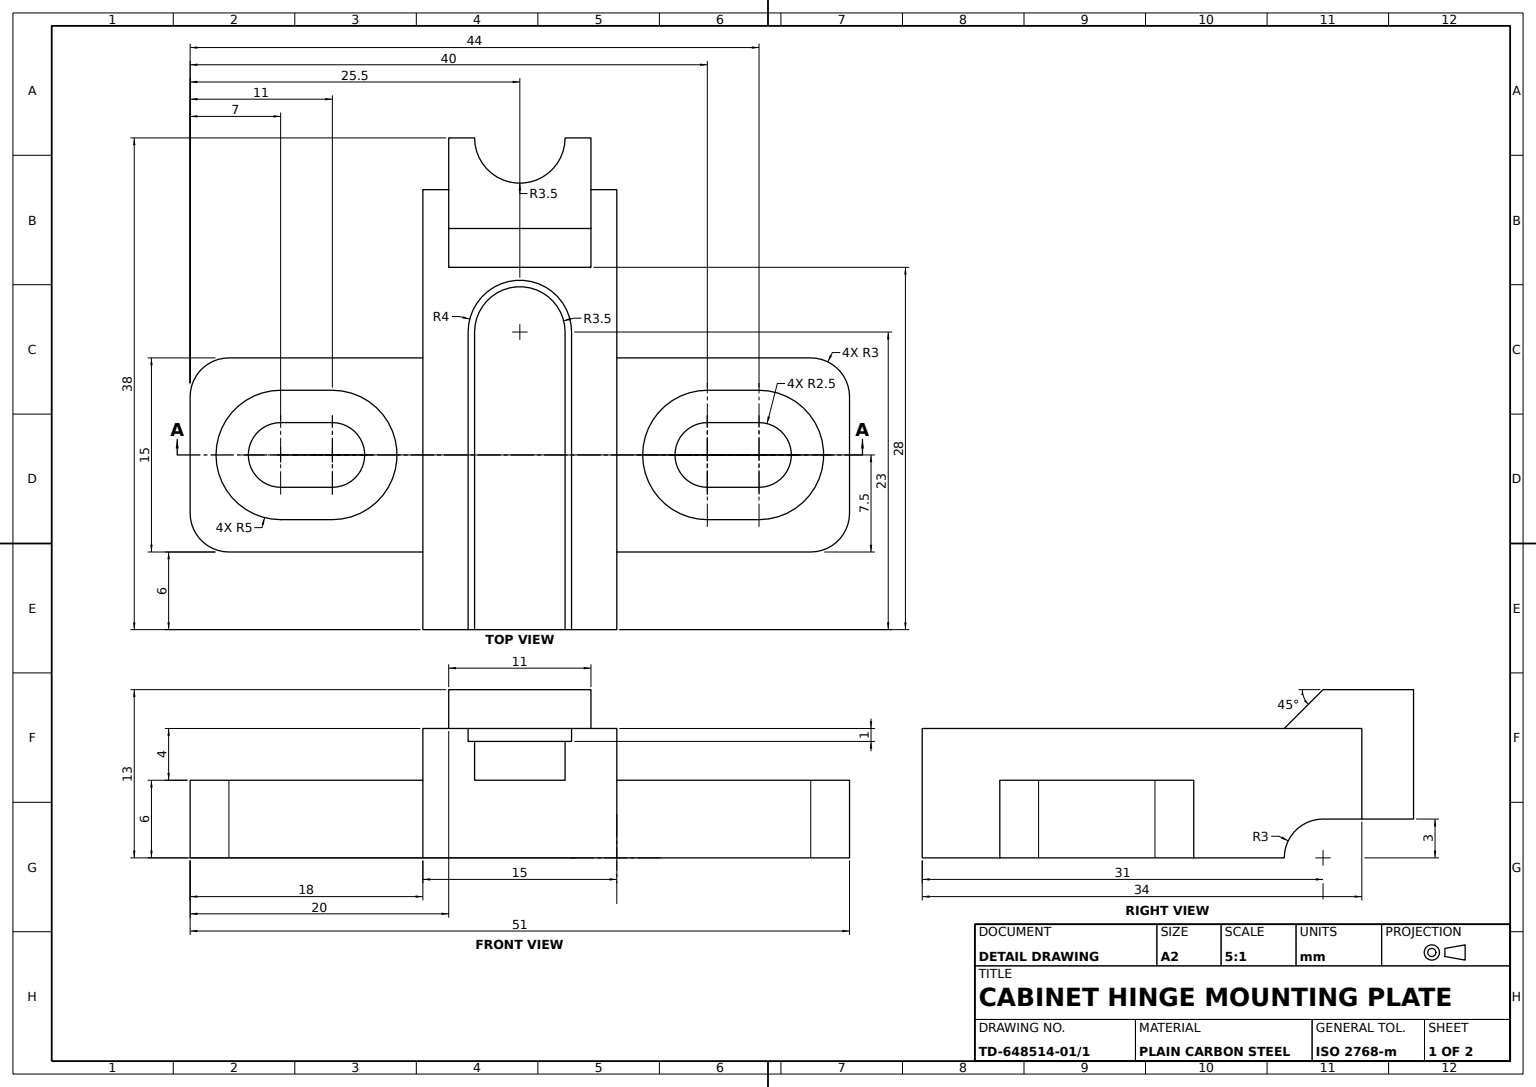
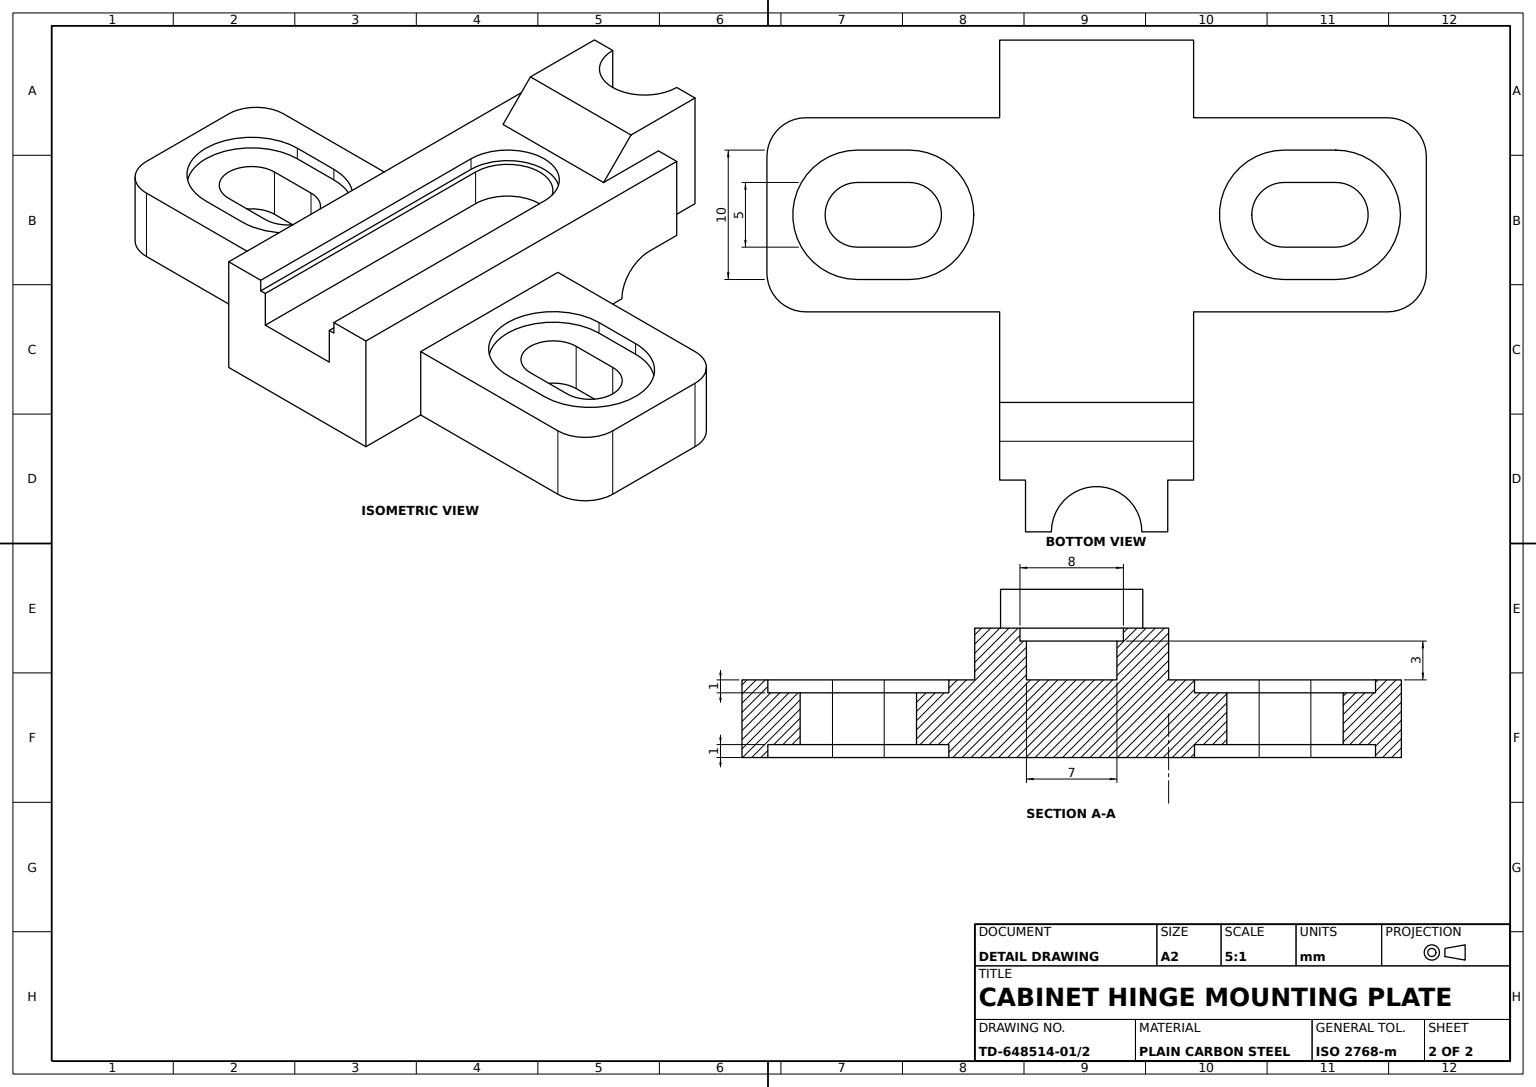
solid
v1 (-5,6,-18.5)
v2 (-5,6,-14.5)
e1 v1 v2 LINE
v3 (-5,5,-14.5)
e2 v3 v2 LINE
v4 (-5,5,-18.5)
e3 v4 v3 LINE
e4 v4 v1 LINE
face PLANE(AX(P(-5,5,-14.5),D(-1,0,0),D(0,0,1))) rev [e1 -e2 -e3 e4]
v5 (-24.5,13,-5.5)
v6 (-24.5,13,-3.5)
e5 v5 v6 LINE
v7 (-24.5,3,-5.5)
e6 v7 v5 LINE
v8 (-24.5,3,-3.5)
e7 v7 v8 LINE
e8 v8 v6 LINE
face PLANE(AX(P(-24.5,3,0),D(-1,0,0),D(0,0,1))) [-e5 -e6 e7 e8]
v9 (4.5,6,-25.5)
v10 (4.5,0,-25.5)
e9 v9 v10 LINE
v11 (-4.5,0,-25.5)
e10 v10 v11 LINE
v12 (-4.5,6,-25.5)
e11 v11 v12 LINE
e12 v9 v12 LINE
face PLANE(AX(P(-7.5,6,-25.5),D(0,0,1),D(1,0,0))) rev [e9 e10 e11 -e12]
v13 (-5,5,14.5)
v14 (5,5,14.5)
e13 v13 v14 CIRCLE(AX(P(0,5,14.5),D(0,-1,0),D(0,0,-1)),5)
v15 (5,6,14.5)
e14 v14 v15 LINE
v16 (-5,6,14.5)
e15 v16 v15 CIRCLE(AX(P(0,6,14.5),D(0,-1,0),D(0,0,-1)),5)
e16 v13 v16 LINE
face CYL(AX(P(0,5,14.5),D(0,1,0),D(0,0,1)),5) rev [e13 e14 -e15 -e16]
v17 (13.5,6,-3.5)
v18 (13.5,9,-3.5)
e17 v17 v18 LINE
v19 (13.5,6,3.5)
e18 v19 v17 LINE
v20 (13.5,9,3.5)
e19 v19 v20 LINE
v21 (13.5,9,4)
e20 v21 v20 LINE
v22 (13.5,10,4)
e21 v21 v22 LINE
v23 (13.5,10,7.5)
e22 v23 v22 LINE
v24 (13.5,0,7.5)
e23 v24 v23 LINE
v25 (13.5,0,-7.5)
e24 v24 v25 LINE
v26 (13.5,10,-7.5)
e25 v25 v26 LINE
v27 (13.5,10,-4)
e26 v27 v26 LINE
v28 (13.5,9,-4)
e27 v28 v27 LINE
e28 v18 v28 LINE
face PLANE(AX(P(13.5,0,7.5),D(1,0,0),D(0,0,-1))) [-e17 -e18 e19 -e20 e21 -e22 -e23 e24 e25 -e26 -e27 -e28]
v29 (-9.5,9,-3.5)
e29 v18 v29 LINE
v30 (-9.5,6,-3.5)
e30 v30 v29 LINE
e31 v17 v30 LINE
face PLANE(AX(P(-9.5,6,-3.5),D(0,0,-1),D(-1,0,0))) rev [e17 e29 -e30 -e31]
v31 (7.5,6,22.5)
v32 (7.5,6,7.5)
e32 v31 v32 LINE
v33 (7.5,0,22.5)
e33 v31 v33 LINE
v34 (7.5,0,7.5)
e34 v33 v34 LINE
e35 v34 v32 LINE
face PLANE(AX(P(7.5,6,-25.5),D(-1,0,0),D(0,0,1))) rev [-e32 e33 e34 e35]
v35 (5,1,-14.5)
v36 (5,0,-14.5)
e36 v35 v36 LINE
v37 (-5,0,-14.5)
e37 v37 v36 CIRCLE(AX(P(0,0,-14.5),D(0,1,0),D(0,0,1)),5)
v38 (-5,1,-14.5)
e38 v38 v37 LINE
e39 v38 v35 CIRCLE(AX(P(0,1,-14.5),D(0,1,0),D(0,0,1)),5)
face CYL(AX(P(0,1,-14.5),D(0,-1,0),D(0,0,-1)),5) rev [e36 -e37 -e38 e39]
v39 (-14.5,10,-5.5)
v40 (-14.5,10,5.5)
e40 v39 v40 LINE
v41 (-17.5,13,-5.5)
e41 v39 v41 LINE
v42 (-17.5,13,5.5)
e42 v41 v42 LINE
e43 v42 v40 LINE
face PLANE(AX(P(-17.5,13,-5.5),D(0.707106781,0.707106781,0),D(0,0,1))) [-e40 e41 e42 e43]
v43 (4.5,0,25.5)
e44 v33 v43 CIRCLE(AX(P(4.5,0,22.5),D(0,-1,0),D(0,0,-1)),3)
v44 (4.5,6,25.5)
e45 v44 v31 CIRCLE(AX(P(4.5,6,22.5),D(0,1,0),D(0,0,-1)),3)
e46 v43 v44 LINE
face CYL(AX(P(4.5,6,22.5),D(0,-1,0),D(0,0,-1)),3) [-e44 -e33 -e45 -e46]
v45 (0,5,-9.5)
v46 (5,5,-14.5)
e47 v45 v46 CIRCLE(AX(P(0,5,-14.5),D(0,1,0),D(0,0,1)),5)
v47 (5,5,-18.5)
e48 v46 v47 LINE
e49 v47 v4 CIRCLE(AX(P(0,5,-18.5),D(0,1,0),D(0,0,1)),5)
e50 v3 v45 CIRCLE(AX(P(0,5,-14.5),D(0,1,0),D(0,0,1)),5)
v48 (-2.5,5,-14.5)
v49 (0,5,-12)
e51 v48 v49 CIRCLE(AX(P(0,5,-14.5),D(0,1,0),D(0,0,1)),2.5)
v50 (-2.5,5,-18.5)
e52 v50 v48 LINE
v51 (2.5,5,-18.5)
e53 v51 v50 CIRCLE(AX(P(0,5,-18.5),D(0,1,0),D(0,0,1)),2.5)
v52 (2.5,5,-14.5)
e54 v52 v51 LINE
e55 v49 v52 CIRCLE(AX(P(0,5,-14.5),D(0,1,0),D(0,0,1)),2.5)
face PLANE(AX(P(0,5,-18.5),D(0,1,0),D(0,0,1))) [e47 e48 e49 e3 e50] [-e51 -e52 -e53 -e54 -e55]
v53 (-9.5,9,4)
e56 v53 v21 LINE
v54 (-9.5,9,3.5)
e57 v54 v20 LINE
e58 v29 v54 CIRCLE(AX(P(-9.5,9,0),D(0,1,0),D(0,0,1)),3.5)
v55 (-9.5,9,-4)
e59 v28 v55 LINE
e60 v55 v53 CIRCLE(AX(P(-9.5,9,0),D(0,1,0),D(0,0,1)),4)
face PLANE(AX(P(-9.5,9,0),D(0,1,0),D(0,0,1))) [e56 e20 -e57 -e58 -e29 e28 e59 e60]
v56 (5,6,18.5)
e61 v15 v56 LINE
v57 (0,6,23.5)
e62 v56 v57 CIRCLE(AX(P(0,6,18.5),D(0,-1,0),D(0,0,-1)),5)
v58 (-5,6,18.5)
e63 v57 v58 CIRCLE(AX(P(0,6,18.5),D(0,-1,0),D(0,0,-1)),5)
e64 v58 v16 LINE
v59 (-7.5,6,7.5)
e65 v32 v59 LINE
v60 (-7.5,6,22.5)
e66 v59 v60 LINE
v61 (-4.5,6,25.5)
e67 v60 v61 CIRCLE(AX(P(-4.5,6,22.5),D(0,1,0),D(0,0,-1)),3)
e68 v61 v44 LINE
face PLANE(AX(P(0,6,0),D(0,-1,0),D(0,0,-1))) rev [e15 e61 e62 e63 e64] [e32 e65 e66 e67 e68 e45]
v62 (-5,1,18.5)
v63 (-5,0,18.5)
e69 v62 v63 LINE
v64 (5,1,18.5)
e70 v64 v62 CIRCLE(AX(P(0,1,18.5),D(0,-1,0),D(0,0,-1)),5)
v65 (5,0,18.5)
e71 v64 v65 LINE
e72 v65 v63 CIRCLE(AX(P(0,0,18.5),D(0,-1,0),D(0,0,-1)),5)
face CYL(AX(P(0,1,18.5),D(0,-1,0),D(0,0,-1)),5) rev [-e69 -e70 e71 e72]
v66 (-5,5,18.5)
e73 v66 v58 LINE
v67 (0,5,23.5)
e74 v67 v57 LINE
e75 v67 v66 CIRCLE(AX(P(0,5,18.5),D(0,-1,0),D(0,0,-1)),5)
face CYL(AX(P(0,5,18.5),D(0,1,0),D(0,0,1)),5) rev [e73 -e63 -e74 e75]
v68 (-7.5,0,-22.5)
e76 v68 v11 CIRCLE(AX(P(-4.5,0,-22.5),D(0,-1,0),D(0,0,-1)),3)
v69 (-7.5,6,-22.5)
e77 v69 v68 LINE
e78 v12 v69 CIRCLE(AX(P(-4.5,6,-22.5),D(0,1,0),D(0,0,-1)),3)
face CYL(AX(P(-4.5,6,-22.5),D(0,-1,0),D(0,0,-1)),3) [-e11 -e76 -e77 -e78]
v70 (7.5,6,-22.5)
e79 v70 v9 CIRCLE(AX(P(4.5,6,-22.5),D(0,1,0),D(0,0,-1)),3)
v71 (-7.5,6,-7.5)
e80 v69 v71 LINE
v72 (7.5,6,-7.5)
e81 v71 v72 LINE
e82 v72 v70 LINE
v73 (5,6,-18.5)
e83 v73 v1 CIRCLE(AX(P(0,6,-18.5),D(0,1,0),D(0,0,1)),5)
v74 (5,6,-14.5)
e84 v74 v73 LINE
v75 (0,6,-9.5)
e85 v75 v74 CIRCLE(AX(P(0,6,-14.5),D(0,1,0),D(0,0,1)),5)
e86 v2 v75 CIRCLE(AX(P(0,6,-14.5),D(0,1,0),D(0,0,1)),5)
face PLANE(AX(P(0,6,0),D(0,-1,0),D(0,0,-1))) rev [e79 e12 e78 e80 e81 e82] [-e1 -e83 -e84 -e85 -e86]
v76 (-24.5,3,3.5)
e87 v76 v8 CIRCLE(AX(P(-24.5,3,0),D(0,1,0),D(0,0,1)),3.5)
v77 (-24.5,13,3.5)
e88 v76 v77 LINE
e89 v77 v6 CIRCLE(AX(P(-24.5,13,0),D(0,1,0),D(0,0,1)),3.5)
face CYL(AX(P(-24.5,3,0),D(0,1,0),D(0,0,1)),3.5) rev [-e87 e88 e89 -e8]
v78 (5,1,14.5)
e90 v78 v64 LINE
v79 (5,0,14.5)
e91 v78 v79 LINE
e92 v79 v65 LINE
face PLANE(AX(P(5,1,14.5),D(1,0,0),D(0,0,-1))) rev [-e90 e91 e92 -e71]
v80 (-4.5,0,25.5)
e93 v61 v80 LINE
e94 v80 v43 LINE
face PLANE(AX(P(7.5,6,25.5),D(0,0,-1),D(-1,0,0))) rev [e46 -e68 e93 e94]
v81 (7.5,0,-7.5)
v82 (7.5,0,-22.5)
e95 v81 v82 LINE
e96 v82 v70 LINE
e97 v72 v81 LINE
face PLANE(AX(P(7.5,6,-25.5),D(-1,0,0),D(0,0,1))) rev [e95 e96 -e82 e97]
v83 (-20.5,10,-7.5)
v84 (-20.5,10,-5.5)
e98 v83 v84 LINE
v85 (-20.5,3,-7.5)
e99 v85 v83 LINE
v86 (-20.5,3,-5.5)
e100 v85 v86 LINE
e101 v86 v84 LINE
face PLANE(AX(P(-20.5,0,0),D(-1,0,0),D(0,0,1))) [-e98 -e99 e100 e101]
v87 (-5,1,-18.5)
e102 v87 v38 LINE
v88 (0,1,-23.5)
e103 v88 v87 CIRCLE(AX(P(0,1,-18.5),D(0,1,0),D(0,0,1)),5)
v89 (5,1,-18.5)
e104 v89 v88 CIRCLE(AX(P(0,1,-18.5),D(0,1,0),D(0,0,1)),5)
e105 v35 v89 LINE
v90 (2.5,1,-14.5)
v91 (2.5,1,-18.5)
e106 v90 v91 LINE
v92 (-2.5,1,-18.5)
e107 v91 v92 CIRCLE(AX(P(0,1,-18.5),D(0,1,0),D(0,0,-1)),2.5)
v93 (-2.5,1,-14.5)
e108 v92 v93 LINE
v94 (0,1,-12)
e109 v93 v94 CIRCLE(AX(P(0,1,-14.5),D(0,1,0),D(0,0,-1)),2.5)
e110 v94 v90 CIRCLE(AX(P(0,1,-14.5),D(0,1,0),D(0,0,-1)),2.5)
face PLANE(AX(P(0,1,-18.5),D(0,-1,0),D(0,0,1))) [-e102 -e103 -e104 -e105 -e39] [e106 e107 e108 e109 e110]
v95 (5,5,18.5)
e111 v95 v56 LINE
e112 v95 v67 CIRCLE(AX(P(0,5,18.5),D(0,-1,0),D(0,0,-1)),5)
face CYL(AX(P(0,5,18.5),D(0,1,0),D(0,0,1)),5) rev [-e111 e112 e74 -e62]
e113 v90 v52 LINE
e114 v91 v51 LINE
face PLANE(AX(P(2.5,-6,-18.5),D(1,0,0),D(0,0,-1))) rev [-e106 e113 e54 -e114]
v96 (-7.5,0,7.5)
e115 v59 v96 LINE
e116 v34 v24 LINE
v97 (-20.5,10,7.5)
e117 v97 v23 LINE
v98 (-20.5,3,7.5)
e118 v98 v97 LINE
v99 (-17.5,3,7.5)
e119 v99 v98 LINE
v100 (-14.5,0,7.5)
e120 v99 v100 CIRCLE(AX(P(-17.5,0,7.5),D(0,0,-1),D(1,0,0)),3)
e121 v100 v96 LINE
face PLANE(AX(P(-9.5,0,7.5),D(0,0,1),D(1,0,0))) [-e115 -e65 -e35 e116 e23 -e117 -e118 -e119 e120 e121]
v101 (-9.5,6,3.5)
e122 v30 v101 CIRCLE(AX(P(-9.5,6,0),D(0,1,0),D(0,0,1)),3.5)
e123 v101 v19 LINE
face PLANE(AX(P(-9.5,6,0),D(0,1,0),D(0,0,1))) [e18 e31 e122 e123]
e124 v66 v13 LINE
face PLANE(AX(P(-5,5,14.5),D(1,0,0),D(0,0,-1))) [e16 -e64 -e73 e124]
e125 v47 v73 LINE
face CYL(AX(P(0,5,-18.5),D(0,1,0),D(0,0,1)),5) rev [-e4 -e49 e125 e83]
v102 (0,0,-23.5)
v103 (-5,0,-18.5)
e126 v102 v103 CIRCLE(AX(P(0,0,-18.5),D(0,1,0),D(0,0,1)),5)
e127 v88 v102 LINE
e128 v87 v103 LINE
face CYL(AX(P(0,1,-18.5),D(0,-1,0),D(0,0,-1)),5) rev [-e126 -e127 e103 e128]
v104 (0,1,21)
v105 (-2.5,1,18.5)
e129 v104 v105 CIRCLE(AX(P(0,1,18.5),D(0,-1,0),D(0,0,-1)),2.5)
v106 (-2.5,5,18.5)
e130 v105 v106 LINE
v107 (0,5,21)
e131 v106 v107 CIRCLE(AX(P(0,5,18.5),D(0,1,0),D(0,0,1)),2.5)
e132 v104 v107 LINE
face CYL(AX(P(0,-6,18.5),D(0,1,0),D(0,0,1)),2.5) rev [e129 e130 e131 -e132]
e133 v45 v75 LINE
face CYL(AX(P(0,5,-14.5),D(0,1,0),D(0,0,1)),5) rev [e2 e86 -e133 -e50]
v108 (5,0,-18.5)
e134 v36 v108 LINE
e135 v108 v102 CIRCLE(AX(P(0,0,-18.5),D(0,1,0),D(0,0,1)),5)
e136 v103 v37 LINE
v109 (0,0,9.5)
e137 v109 v79 CIRCLE(AX(P(0,0,14.5),D(0,-1,0),D(0,0,-1)),5)
v110 (-5,0,14.5)
e138 v110 v109 CIRCLE(AX(P(0,0,14.5),D(0,-1,0),D(0,0,-1)),5)
e139 v63 v110 LINE
v111 (-7.5,0,22.5)
e140 v96 v111 LINE
v112 (-14.5,0,-7.5)
e141 v112 v100 LINE
v113 (-7.5,0,-7.5)
e142 v113 v112 LINE
e143 v68 v113 LINE
e144 v10 v82 CIRCLE(AX(P(4.5,0,-22.5),D(0,-1,0),D(0,0,-1)),3)
e145 v25 v81 LINE
e146 v80 v111 CIRCLE(AX(P(-4.5,0,22.5),D(0,-1,0),D(0,0,-1)),3)
face PLANE(AX(P(0,0,0),D(0,-1,0),D(0,0,-1))) [e134 e135 e126 e136 e37] [-e72 -e92 -e137 -e138 -e139] [-e140 -e121 -e141 -e142 -e143 e76 -e10 e144 -e95 -e145 -e24 -e116 -e34 e44 -e94 e146]
v114 (-24.5,3,5.5)
e147 v76 v114 LINE
v115 (-24.5,13,5.5)
e148 v114 v115 LINE
e149 v77 v115 LINE
face PLANE(AX(P(-24.5,3,0),D(-1,0,0),D(0,0,1))) [-e88 e147 e148 -e149]
v116 (-2.5,1,14.5)
v117 (2.5,1,14.5)
e150 v116 v117 CIRCLE(AX(P(0,1,14.5),D(0,-1,0),D(0,0,-1)),2.5)
v118 (2.5,5,14.5)
e151 v117 v118 LINE
v119 (-2.5,5,14.5)
e152 v118 v119 CIRCLE(AX(P(0,5,14.5),D(0,1,0),D(0,0,1)),2.5)
e153 v116 v119 LINE
face CYL(AX(P(0,-6,14.5),D(0,1,0),D(0,0,1)),2.5) rev [e150 e151 e152 -e153]
v120 (-17.5,3,-7.5)
e154 v85 v120 LINE
e155 v120 v99 LINE
v121 (-20.5,3,5.5)
e156 v121 v98 LINE
e157 v114 v121 LINE
e158 v86 v7 LINE
face PLANE(AX(P(0,3,0),D(0,1,0),D(0,0,1))) rev [-e100 e154 e155 e119 -e156 -e157 -e147 e87 -e7 -e158]
e159 v46 v74 LINE
face PLANE(AX(P(5,5,-14.5),D(1,0,0),D(0,0,-1))) rev [e84 -e125 -e48 e159]
e160 v41 v5 LINE
e161 v84 v39 LINE
face PLANE(AX(P(0,3,-5.5),D(0,0,-1),D(-1,0,0))) [-e160 -e41 -e161 -e101 e158 e6]
v122 (0,1,9.5)
e162 v122 v78 CIRCLE(AX(P(0,1,14.5),D(0,-1,0),D(0,0,-1)),5)
e163 v122 v109 LINE
face CYL(AX(P(0,1,14.5),D(0,-1,0),D(0,0,-1)),5) rev [-e91 -e162 e163 e137]
face PLANE(AX(P(-5,1,-14.5),D(1,0,0),D(0,0,-1))) [-e128 e102 e38 -e136]
v123 (2.5,1,18.5)
e164 v123 v104 CIRCLE(AX(P(0,1,18.5),D(0,-1,0),D(0,0,-1)),2.5)
e165 v117 v123 LINE
e166 v105 v116 LINE
v124 (-5,1,14.5)
e167 v62 v124 LINE
e168 v124 v122 CIRCLE(AX(P(0,1,14.5),D(0,-1,0),D(0,0,-1)),5)
face PLANE(AX(P(0,1,18.5),D(0,-1,0),D(0,0,-1))) [-e129 -e164 -e165 -e150 -e166] [e162 e90 e70 e167 e168]
e169 v94 v49 LINE
face CYL(AX(P(0,-6,-14.5),D(0,1,0),D(0,0,1)),2.5) rev [-e113 -e110 e169 e55]
e170 v92 v50 LINE
face CYL(AX(P(0,-6,-18.5),D(0,1,0),D(0,0,1)),2.5) rev [e53 -e170 -e107 e114]
e171 v112 v120 CIRCLE(AX(P(-17.5,0,-7.5),D(0,0,1),D(-1,0,0)),3)
face CYL(AX(P(-17.5,0,0),D(0,0,-1),D(-1,0,0)),3) rev [-e171 e141 -e120 -e155]
e172 v124 v110 LINE
face PLANE(AX(P(-5,1,14.5),D(-1,0,0),D(0,0,1))) rev [e139 -e172 -e167 e69]
e173 v14 v95 LINE
face PLANE(AX(P(5,5,14.5),D(-1,0,0),D(0,0,1))) [-e61 -e14 e173 e111]
e174 v93 v48 LINE
face CYL(AX(P(0,-6,-14.5),D(0,1,0),D(0,0,1)),2.5) rev [-e109 e174 e51 -e169]
v125 (2.5,5,18.5)
e175 v107 v125 CIRCLE(AX(P(0,5,18.5),D(0,1,0),D(0,0,1)),2.5)
e176 v119 v106 LINE
e177 v125 v118 LINE
face PLANE(AX(P(0,5,18.5),D(0,1,0),D(0,0,-1))) [-e124 -e75 -e112 -e173 -e13] [-e175 -e131 -e176 -e152 -e177]
face PLANE(AX(P(-2.5,-6,14.5),D(-1,0,0),D(0,0,1))) rev [-e130 e166 e153 e176]
face CYL(AX(P(4.5,6,-22.5),D(0,-1,0),D(0,0,-1)),3) [-e9 -e79 -e96 -e144]
e178 v101 v54 LINE
face PLANE(AX(P(13.5,6,3.5),D(0,0,1),D(1,0,0))) rev [-e19 -e123 e178 e57]
face CYL(AX(P(0,1,14.5),D(0,-1,0),D(0,0,-1)),5) rev [e138 -e163 -e168 e172]
v126 (-9.5,10,4)
e179 v126 v22 LINE
e180 v53 v126 LINE
face PLANE(AX(P(13.5,9,4),D(0,0,1),D(1,0,0))) rev [e179 -e21 -e56 e180]
e181 v113 v71 LINE
e182 v26 v83 LINE
face PLANE(AX(P(13.5,0,-7.5),D(0,0,-1),D(-1,0,0))) [e145 -e97 -e81 -e181 e142 e171 -e154 e99 -e182 -e25]
e183 v115 v42 LINE
face PLANE(AX(P(0,13,0),D(0,1,0),D(0,0,1))) [-e42 e160 e5 -e89 e149 e183]
e184 v111 v60 LINE
face CYL(AX(P(-4.5,6,22.5),D(0,-1,0),D(0,0,-1)),3) [-e93 -e67 -e184 -e146]
v127 (-20.5,10,5.5)
e185 v127 v40 LINE
e186 v121 v127 LINE
face PLANE(AX(P(0,3,5.5),D(0,0,1),D(1,0,0))) [e185 -e43 -e183 -e148 e157 e186]
e187 v89 v108 LINE
face CYL(AX(P(0,1,-18.5),D(0,-1,0),D(0,0,-1)),5) rev [-e187 e104 e127 -e135]
v128 (-9.5,10,-4)
e188 v55 v128 LINE
e189 v128 v126 CIRCLE(AX(P(-9.5,10,0),D(0,1,0),D(0,0,1)),4)
face CYL(AX(P(-9.5,9,0),D(0,1,0),D(0,0,1)),4) rev [-e60 e188 e189 -e180]
face PLANE(AX(P(-7.5,6,0),D(1,0,0),D(0,0,-1))) rev [e77 e143 e181 -e80]
e190 v123 v125 LINE
face CYL(AX(P(0,-6,18.5),D(0,1,0),D(0,0,1)),2.5) rev [e175 -e190 e164 e132]
face PLANE(AX(P(-2.5,-6,-18.5),D(-1,0,0),D(0,0,1))) rev [-e174 -e108 e170 e52]
face PLANE(AX(P(-7.5,6,0),D(1,0,0),D(0,0,-1))) rev [e140 e184 -e66 e115]
face CYL(AX(P(-9.5,6,0),D(0,1,0),D(0,0,1)),3.5) rev [e30 e58 -e178 -e122]
face PLANE(AX(P(5,1,-14.5),D(-1,0,0),D(0,0,1))) [-e36 e105 e187 -e134]
face CYL(AX(P(0,5,-14.5),D(0,1,0),D(0,0,1)),5) rev [-e159 -e47 e133 e85]
e191 v27 v128 LINE
e192 v127 v97 LINE
face PLANE(AX(P(0,10,0),D(0,1,0),D(0,0,1))) [-e191 e26 e182 e98 e161 e40 -e185 e192 e117 e22 -e179 -e189]
face PLANE(AX(P(-9.5,9,-4),D(0,0,-1),D(-1,0,0))) rev [-e188 -e59 e27 e191]
face PLANE(AX(P(2.5,-6,14.5),D(1,0,0),D(0,0,-1))) rev [e177 -e151 e165 e190]
face PLANE(AX(P(-20.5,0,0),D(-1,0,0),D(0,0,1))) [-e186 e156 e118 -e192]
